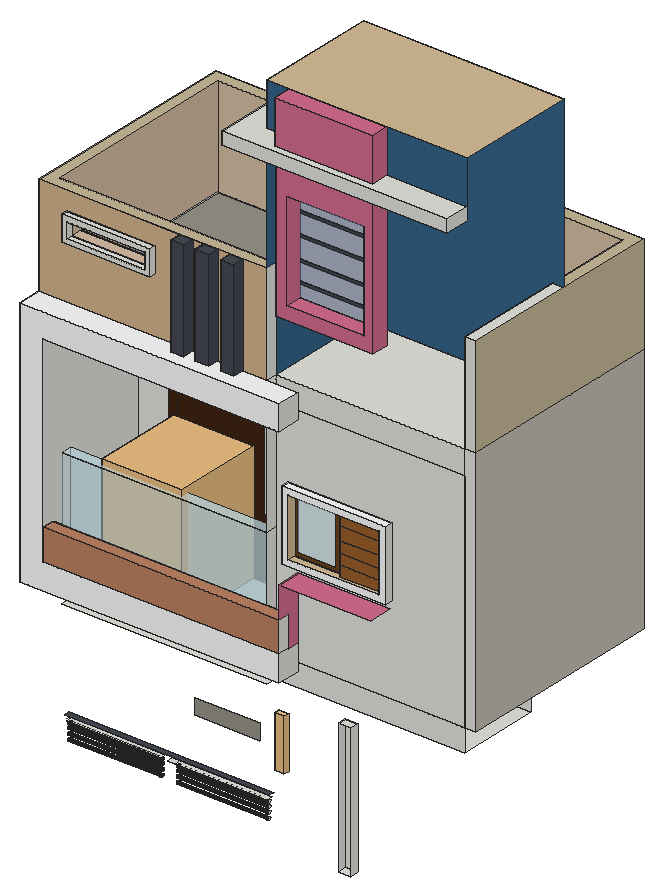
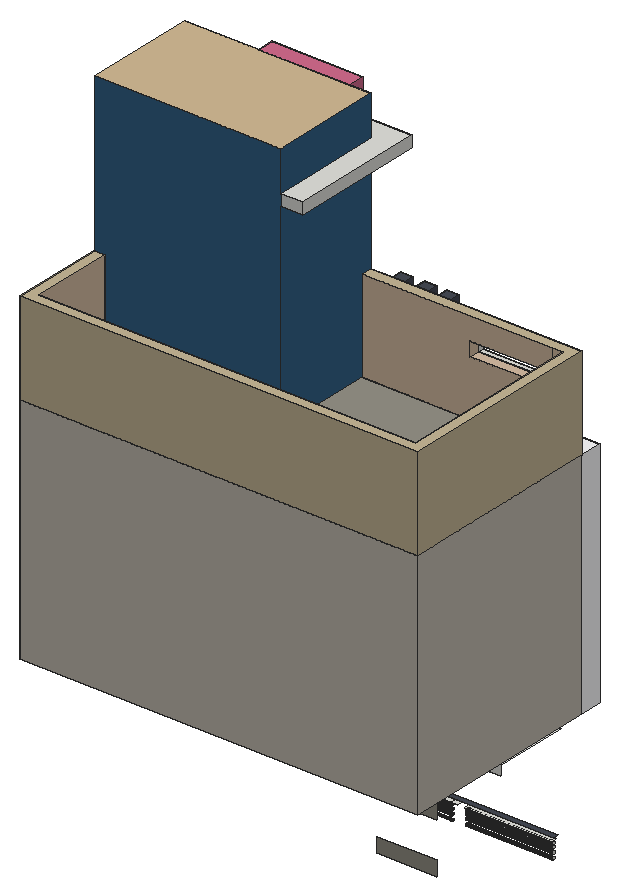
# SketchUp Ruby script. Lengths in inches.
U = 1.inch
M = Sketchup.active_model
def pt(a) = Geom::Point3d.new(a.map { |v| v * U })
def face(e, loops, mat)
  f = e.add_face(loops[0].map { |a| pt(a) })
  loops[1..].each { |l| e.add_face(l.map { |a| pt(a) }).erase! }
  f.material = f.back_material = mat if mat
  f
end
# faces: each face lists its corners as indices into pts; further lists are holes
def faces(e, pts, list, mat = nil) = list.each { |f| face(e, (f[0].is_a?(Array) ? f : [f]).map { |l| l.map { |i| pts[i] } }, mat) }
# xy, xz, yz: faces in a plane at the given z, y or x. An outline is a flat list of corners, or four numbers for a rectangle; further outlines are holes
def ring(l) = l.size == 4 ? [[l[0], l[1]], [l[2], l[1]], [l[2], l[3]], [l[0], l[3]]] : l.each_slice(2).to_a
def flat(e, list, mat, &to3) = list.each { |f| face(e, (f[0].is_a?(Array) ? f : [f]).map { |l| ring(l).map { |u, v| to3.(u, v) } }, mat) }
def xy(e, z, list, mat = nil) = flat(e, list, mat) { |x, y| [x, y, z] }
def xz(e, y, list, mat = nil) = flat(e, list, mat) { |x, z| [x, y, z] }
def yz(e, x, list, mat = nil) = flat(e, list, mat) { |y, z| [x, y, z] }
def lines(e, pts, list) = list.each { |a, b| e.add_line(pt(pts[a]), pt(pts[b])) }
# prism: a flat outline (further loops are holes) pulled along v
def prism(e, loops, v, mat = nil)
  f = face(e, loops, mat); d = Geom::Vector3d.new(v.map { |x| x * U })
  f.pushpull(f.normal.samedirection?(d) ? d.length : -d.length)
end
def box(e, o, s, mat = nil) = prism(e, [[o, [o[0] + s[0], o[1], o[2]], [o[0] + s[0], o[1] + s[1], o[2]], [o[0], o[1] + s[1], o[2]]]], [0, 0, s[2]], mat)
def at(x, y, z, deg = 0) = Geom::Transformation.translation(pt([x, y, z])) * Geom::Transformation.rotation(ORIGIN, Z_AXIS, deg.degrees)
def axes(o, x, y, z) = Geom::Transformation.new([*x, 0, *y, 0, *z, 0, *pt(o).to_a, 1])
def part(name) = M.definitions.add(name)
# library, detail: a bought-in or finely detailed component or shape, given as its bounding box
def library(name, o, s) = part(name).tap { |d| box(d.entities, o, s) }
def detail(e, o, s) = box(e.add_group.entities, o, s)
def put(e, d, t, mat = nil) = e.add_instance(d, t).tap { |i| i.material = mat if mat }
def group(e, t, mat = nil) = e.add_group.tap { |g| g.transformation = t; g.material = mat if mat }.entities
root = M.entities
M.materials.add("[0001_PaleVioletRed]").color = [211, 108, 142]
M.materials.add("[0035_Tan]").color = [210, 180, 140]
M.materials.add("[0100_SteelBlue]").color = [53, 99, 137]
M.materials.add("[Field Rectangle Tile]").color = [196, 189, 179]
M.materials.add("[Formica Beige]").color = [211, 187, 149]
M.materials.add("[Formica Graystone]").color = [149, 146, 135]
M.materials.add("[Formica Laminate Dark]").color = [70, 74, 84]
M.materials.add("[Formica Laminate Light]").color = [213, 189, 164]
M.materials.add("[Modern Siding]").color = [188, 130, 98]
M.materials.add("[Polished Concrete New]").color = [200, 200, 203]
M.materials.add("[Quartz Light Brown]").color = [199, 184, 152]
M.materials.add("[Quartz Light Grey]").color = [251, 251, 252]
M.materials.add("[Terrazzo Tile Light]").color = [219, 217, 210]
M.materials.add("[Translucent Glass Safety]").color = [204, 235, 244]
M.materials["[Translucent Glass Safety]"].alpha = 0.5
M.materials.add("[Translucent Glass Sky Reflection]").color = [126, 138, 183]
M.materials["[Translucent Glass Sky Reflection]"].alpha = 0.52
M.materials.add("[Window Covering 02]").color = [199, 178, 115]
M.materials.add("[Wood Cherry Original]").color = [96, 54, 26]
M.materials.add("[Wood Floor Dark]").color = [153, 94, 42]
M.materials.add("[Wood Floor Parquet]").color = [107, 65, 28]
M.materials.add("[Wood Veneer 01]").color = [63, 37, 19]
c1 = library("0 0 1",[0.77,0,0],[4.67,38.51,12])
c2 = library("chau cay",[-24.34,-109.24,0],[56.46,62.58,79.69])
xy(root,57.97,[[248.98,105.92,254.98,109.98]])
xy(root,67.58,[[108.27,118.87,153.22,121.64],[156.73,118.87,160.24,121.64],[160.24,118.87,204.4,121.64]])
xy(root,69.75,[[107.21,118.87,205.34,121.64]],"[Formica Laminate Dark]")
xy(root,118.16,[[107.21,117.35,107.21,162.72,296.05,162.72,296.05,122.78,205.34,122.78,205.34,117.35]])
xy(root,121.72,[[248.98,105.92,254.98,109.98]])
xy(root,129,[[96.16,105.92,101.58,117.35],[101.58,105.92,205.34,117.35],[205.34,105.92,220.625,117.35],[96.16,117.35,96.16,223.51,301.48,223.51,301.48,122.78,296.05,122.78,296.05,218.08,101.58,218.08,101.58,162.72,107.21,162.72,107.21,122.78,101.58,122.78,101.58,117.35],[101.58,117.35,205.34,122.78],
  [107.21,122.78,296.05,162.72],[101.58,162.72,296.05,170.43],[101.58,170.43,296.05,218.08]])
xy(root,141.375,[[107.21,105.92,220.625,111.64],[107.21,111.64,220.625,117.35],[107.21,117.35,205.34,122.78]])
xy(root,156.32,[[107.21,105.92,220.625,111.64]],"[Modern Siding]")
xy(root,162.92,[[195.11,162.72,264.3,170.43]])
xy(root,171.19,[[220.625,105.92,264.66,117.35]],"[0001_PaleVioletRed]")
xy(root,175.07,[[215.78,113.67,265.4,117.35]])
xy(root,178.04,[[241.96,115.6,262.43,117.35]])
xy(root,178.04,[[218.75,113.67,262.43,113.67,262.43,115.6,241.96,115.6,241.96,117.35,218.75,117.35]],"[Formica Beige]")
xy(root,183.1,[[241.96,115.6,262.43,117.35]])
xy(root,183.25,[[107.21,117.35,205.34,122.78]],"[Translucent Glass Safety]")
xy(root,188.16,[[241.96,115.6,262.43,117.35]])
xy(root,193.62,[[241.96,115.6,262.43,117.35]])
xy(root,199.79,[[241.96,115.6,262.43,117.35]])
xy(root,205.7,[[241.96,115.6,262.43,117.35]])
xy(root,205.7,[[218.75,113.67,218.75,117.35,241.96,117.35,241.96,115.6,262.43,115.6,262.43,113.67]],"[Formica Beige]")
xy(root,208.67,[[215.78,113.67,265.4,117.35]],"[Quartz Light Grey]")
xy(root,232.11,[[195.11,162.72,264.3,170.43]])
xy(root,237.17,[[107.21,105.92,205.34,117.35],[205.34,105.92,220.625,117.35],[107.21,117.35,205.34,122.78],[107.21,122.78,296.05,162.72]])
xy(root,239.2,[[101.58,170.43,296.05,218.08]])
xy(root,249,[[163.85,111.98,170.19,117.35],[175.41,111.98,181.76,117.35],[187.73,111.98,194.07,117.35],[96.16,117.35,96.16,223.51,301.48,223.51,301.48,122.78,296.05,122.78,296.05,218.08,101.58,218.08,101.58,117.35],[101.58,117.35,205.34,122.78],
  [205.34,122.78,296.05,175.59]])
xy(root,249,[[101.58,122.78,205.34,122.78,205.34,175.59,296.05,175.59,296.05,218.08,101.58,218.08]],"[Formica Graystone]")
xy(root,249,[[96.16,105.92,220.625,105.92,220.625,117.35,194.07,117.35,194.07,111.98,187.73,111.98,187.73,117.35,181.76,117.35,181.76,111.98,175.41,111.98,175.41,117.35,170.19,117.35,170.19,111.98,163.85,111.98,163.85,117.35,96.16,117.35]],"[Quartz Light Grey]")
xy(root,275.81,[[109.44,114.48,151.75,117.35]])
xy(root,278.13,[[111.77,114.48,149.43,117.35]])
xy(root,278.13,[[111.77,117.35,149.43,122.78]],"[Formica Laminate Light]")
xy(root,284.16,[[216.72,108.73,263.15,117.35]],"[0001_PaleVioletRed]")
xy(root,285.55,[[111.77,114.48,149.43,117.35]])
xy(root,285.55,[[111.77,117.35,149.43,122.78]],"[Formica Laminate Light]")
xy(root,287.87,[[109.44,114.48,151.75,117.35]])
xy(root,290.43,[[221.94,108.73,258.81,116.79]],"[0001_PaleVioletRed]")
xy(root,297,[[296.05,122.78,301.48,175.59]])
xy(root,297,[[163.85,111.98,170.19,117.35],[175.41,111.98,181.76,117.35],[187.73,111.98,194.07,117.35]],"[Formica Laminate Dark]")
xy(root,297,[[96.16,117.35,205.34,117.35,205.34,122.78,101.58,122.78,101.58,218.08,296.05,218.08,296.05,175.59,301.48,175.59,301.48,223.51,96.16,223.51]],"[Quartz Light Brown]")
xy(root,337.68,[[221.94,108.73,258.81,116.79]],"[0001_PaleVioletRed]")
xy(root,351.35,[[193.71,105.1,193.71,175.59,205.34,175.59,205.34,117.35,216.72,117.35,216.72,108.73,263.15,108.73,263.15,117.35,266.37,117.35,266.37,114.04,301.48,114.04,301.48,105.1],[216.72,108.73,263.15,117.35],[266.37,114.04,301.48,117.35]])
xy(root,357.29,[[193.71,105.1,301.48,105.1,301.48,117.35,263.15,117.35,263.15,108.73,216.08,108.73,216.08,117.35,205.34,117.35,205.34,175.59,193.71,175.59],[216.08,108.73,263.15,117.35]])
xy(root,378.0625,[[216.08,108.73,263.15,117.35]],"[0001_PaleVioletRed]")
xy(root,378.0625,[[205.34,117.35,301.48,175.59]],"[Formica Beige]")
xz(root,105.1,[[193.71,351.35,301.48,357.29]])
xz(root,105.92,[[107.21,141.375,220.625,156.32]],"[Modern Siding]")
xz(root,105.92,[[96.16,129,220.625,129,220.625,141.375,107.21,141.375,107.21,237.17,220.625,237.17,220.625,249,96.16,249]],"[Quartz Light Grey]")
xz(root,108.73,[[[216.72,284.16,263.15,351.35],[221.94,290.43,258.81,337.68]],[216.08,357.29,263.15,378.0625]],"[0001_PaleVioletRed]")
xz(root,109.98,[[248.98,57.97,254.98,121.72]])
xz(root,111.64,[[107.21,141.375,220.625,156.32]])
xz(root,111.98,[[163.85,249,170.19,297],[175.41,249,181.76,297],[187.73,249,194.07,297]],"[Formica Laminate Dark]")
xz(root,113.67,[[[215.78,175.07,265.4,208.67],[218.75,178.04,262.43,205.7]]],"[Quartz Light Grey]")
xz(root,114.48,[[[109.44,275.81,151.75,287.87],[111.77,278.13,149.43,285.55]]])
xz(root,115.6,[[241.96,178.04,262.43,183.1],[241.96,183.1,262.43,188.16],[241.96,188.16,262.43,193.62],[241.96,193.62,262.43,199.79],[241.96,199.79,262.43,205.7]],"[Wood Floor Dark]")
xz(root,116.79,[[221.94,296.5,258.81,297.76],[221.94,306.0625,258.81,307.32],[221.94,316.75,258.81,318.01],[221.94,327.125,258.81,328.38]],"[Formica Laminate Dark]")
xz(root,116.79,[[221.94,290.43,258.81,296.5],[221.94,297.76,258.81,306.0625],[221.94,307.32,258.81,316.75],[221.94,318.01,258.81,327.125],[221.94,328.38,258.81,337.68]],"[Translucent Glass Sky Reflection]")
xz(root,117.35,[[[215.78,175.07,265.4,208.67],[218.75,178.04,262.43,205.7]],[241.96,178.04,262.43,183.1],[241.96,183.1,262.43,188.16],[241.96,188.16,262.43,193.62],[241.96,193.62,262.43,199.79],
  [241.96,199.79,262.43,205.7],[163.85,249,170.19,297],[175.41,249,181.76,297],[187.73,249,194.07,297],[[109.44,275.81,151.75,287.87],[111.77,278.13,149.43,285.55]],
  [216.72,284.16,263.15,351.35],[216.08,357.29,263.15,378.0625]])
xz(root,117.35,[[[96.16,249,163.85,297],[109.44,275.81,151.75,287.87]],[170.19,249,175.41,297],[181.76,249,187.73,297],[194.07,249,205.34,297]],"[0035_Tan]")
xz(root,117.35,[[205.34,357.29,216.08,378.0625],[263.15,357.29,301.48,378.0625]],"[0100_SteelBlue]")
xz(root,117.35,[[240.59,178.04,241.96,205.7]],"[Formica Laminate Dark]")
xz(root,117.35,[[107.21,141.375,205.34,183.25],[220.59,179.88,238.75,203.85]],"[Translucent Glass Safety]")
xz(root,117.35,[[[218.75,178.04,240.59,205.7],[220.59,179.88,238.75,203.85]]],"[Wood Floor Parquet]")
xz(root,122.78,[[205.34,118.16,296.05,129],[107.21,129,205.34,141.375],[205.34,129,296.05,237.17],[296.05,129,301.48,249],[107.21,237.17,205.34,249],
  [205.34,237.17,296.05,249],[296.05,249,301.48,297]])
xz(root,122.78,[[101.58,249,107.21,297],[[107.21,249,205.34,297],[111.77,278.13,149.43,285.55]]],"[Formica Laminate Light]")
xz(root,122.78,[[107.21,141.375,205.34,183.25]],"[Translucent Glass Safety]")
xz(root,162.72,[[101.58,118.16,296.05,129],[[107.21,129,121.5625,129,121.5625,232.125,181,232.125,181,129,296.05,129,296.05,237.17,107.21,237.17],[195.11,162.92,264.3,232.11]]])
xz(root,162.72,[[134.59,60.26,166.02,67.7],[134.59,86.26,166.02,93.7],[131.36,156.37,163.17,163.24],[131.36,178.99,163.17,185.87],[131.36,202.49,163.17,209.37]],"[Formica Graystone]")
xz(root,162.72,[[167.92,157.88,170.35,202.19]],"[Terrazzo Tile Light]")
xz(root,162.72,[[199.8,167.62,226.2,227.42],[230.11,167.62,259.61,227.42]],"[Window Covering 02]")
xz(root,162.72,[[[195.11,162.92,264.3,232.11],[199.8,167.62,259.61,227.42]],[226.2,167.62,230.11,227.42]],"[Wood Cherry Original]")
xz(root,162.72,[[[121.5625,129,181,232.125],[126.22,133.65,176.35,227.47]],[[126.22,133.65,176.35,227.47],[131.36,202.49,163.17,209.37],[131.36,156.37,163.17,163.24],[131.36,178.99,163.17,185.87],[167.92,157.88,170.35,202.19]]],"[Wood Veneer 01]")
xz(root,170.43,[[[101.58,129,296.05,239.2],[195.11,162.92,264.3,232.11]]])
xz(root,175.59,[[193.71,351.35,205.34,357.29]])
xz(root,175.59,[[205.34,249,205.34,378.0625,301.48,378.0625,301.48,297,296.05,297,296.05,249]],"[0100_SteelBlue]")
xz(root,218.08,[[101.58,129,296.05,239.2],[101.58,239.2,296.05,249]])
xz(root,218.08,[[101.58,249,296.05,297]],"[Formica Laminate Light]")
xz(root,223.51,[[96.16,129,301.48,249]],"[Field Rectangle Tile]")
xz(root,223.51,[[96.16,249,301.48,297]],"[Quartz Light Brown]")
yz(root,96.16,[[117.35,129,223.51,249]],"[Field Rectangle Tile]")
yz(root,96.16,[[117.35,249,223.51,297]],"[Quartz Light Brown]")
yz(root,96.16,[[105.92,129,117.35,249]],"[Quartz Light Grey]")
yz(root,101.58,[[162.72,129,170.43,249],[170.43,129,218.08,239.2],[170.43,239.2,218.08,249]])
yz(root,101.58,[[122.78,249,218.08,297]],"[Formica Laminate Light]")
yz(root,107.21,[[122.78,129,162.72,129,162.72,237.17,105.92,237.17,105.92,156.32,111.64,156.32,111.64,141.375,117.35,141.375,117.35,183.25,122.78,183.25],[105.92,141.375,111.64,156.32],[117.35,141.375,122.78,183.25]])
yz(root,108.27,[[120.22,58.6,120.06,58.62,119.91,58.68,119.78,58.78,119.68,58.91,119.61,59.0625,119.59,59.22,119.61,59.38,119.68,59.54,119.78,59.66,119.91,59.76,120.06,59.83,120.22,59.85,120.38,59.83,120.53,59.76,120.66,59.66,120.76,59.54,120.82,59.38,120.84,59.22,120.82,59.0625,120.76,58.91,120.66,58.78,120.53,58.68,120.38,58.62],[120.22,61.16,120.06,61.18,119.91,61.24,119.78,61.34,119.68,61.47,119.61,61.625,119.59,61.79,119.61,61.95,119.68,62.1,119.78,62.23,119.91,62.33,120.06,62.39,120.22,62.41,120.38,62.39,120.53,62.33,120.66,62.23,120.76,62.1,120.82,61.95,120.84,61.79,120.82,61.625,120.76,61.47,120.66,61.34,120.53,61.24,120.38,61.18],[120.22,63.72,120.06,63.74,119.91,63.81,119.78,63.91,119.68,64.04,119.61,64.1875,119.59,64.35,119.61,64.51,119.68,64.66,119.78,64.79,119.91,64.89,120.06,64.95,120.22,64.97,120.38,64.95,120.53,64.89,120.66,64.79,120.76,64.66,120.82,64.51,120.84,64.35,120.82,64.1875,120.76,64.04,120.66,63.91,120.53,63.81,120.38,63.74],[120.22,65.6,120.06,65.62,119.91,65.68,119.78,65.78,119.68,65.91,119.61,66.0625,119.59,66.22,119.61,66.38,119.68,66.54,119.78,66.66,119.91,66.76,120.06,66.83,120.22,66.85,120.38,66.83,120.53,66.76,120.66,66.66,120.76,66.54,120.82,66.38,120.84,66.22,120.82,66.0625,120.76,65.91,120.66,65.78,120.53,65.68,120.38,65.62]])
yz(root,109.44,[[114.48,275.81,117.35,287.87]])
yz(root,111.77,[[114.48,278.13,117.35,285.55]])
yz(root,111.77,[[117.35,278.13,122.78,285.55]],"[Formica Laminate Light]")
yz(root,149.43,[[114.48,278.13,117.35,285.55]])
yz(root,149.43,[[117.35,278.13,122.78,285.55]],"[Formica Laminate Light]")
yz(root,151.75,[[114.48,275.81,117.35,287.87]])
yz(root,163.85,[[111.98,249,117.35,297]],"[Formica Laminate Dark]")
yz(root,170.19,[[111.98,249,117.35,297]],"[Formica Laminate Dark]")
yz(root,175.41,[[111.98,249,117.35,297]],"[Formica Laminate Dark]")
yz(root,181.76,[[111.98,249,117.35,297]],"[Formica Laminate Dark]")
yz(root,187.73,[[111.98,249,117.35,297]],"[Formica Laminate Dark]")
yz(root,193.71,[[105.1,351.35,175.59,357.29]])
yz(root,194.07,[[111.98,249,117.35,297]],"[Formica Laminate Dark]")
yz(root,195.11,[[162.72,162.92,170.43,232.11]])
yz(root,204.4,[[120.29,58.16,120.45,58.1875,120.6,58.25,120.73,58.35,120.83,58.48,120.89,58.63,120.91,58.79,120.89,58.95,120.83,59.1,120.73,59.23,120.6,59.33,120.45,59.39,120.29,59.41,120.13,59.39,119.98,59.33,119.85,59.23,119.75,59.1,119.6875,58.95,119.66,58.79,119.6875,58.63,119.75,58.48,119.85,58.35,119.98,58.25,120.13,58.1875],[120.29,60.85,120.45,60.875,120.6,60.9375,120.73,61.04,120.83,61.16,120.89,61.32,120.91,61.48,120.89,61.64,120.83,61.79,120.73,61.92,120.6,62.02,120.45,62.08,120.29,62.1,120.13,62.08,119.98,62.02,119.85,61.92,119.75,61.79,119.6875,61.64,119.66,61.48,119.6875,61.32,119.75,61.16,119.85,61.04,119.98,60.9375,120.13,60.875],[120.29,63.23,120.45,63.25,120.6,63.3125,120.73,63.41,120.83,63.54,120.89,63.69,120.91,63.85,120.89,64.01,120.83,64.16,120.73,64.29,120.6,64.39,120.45,64.46,120.29,64.48,120.13,64.46,119.98,64.39,119.85,64.29,119.75,64.16,119.6875,64.01,119.66,63.85,119.6875,63.69,119.75,63.54,119.85,63.41,119.98,63.3125,120.13,63.25],[120.29,65.54,120.45,65.5625,120.6,65.625,120.73,65.72,120.83,65.85,120.89,66,120.91,66.16,120.89,66.33,120.83,66.48,120.73,66.61,120.6,66.71,120.45,66.77,120.29,66.79,120.13,66.77,119.98,66.71,119.85,66.61,119.75,66.48,119.6875,66.33,119.66,66.16,119.6875,66,119.75,65.85,119.85,65.72,119.98,65.625,120.13,65.5625]])
yz(root,205.34,[[117.35,141.375,122.78,183.25],[117.35,183.25,122.78,237.17],[117.35,249,122.78,297]])
yz(root,205.34,[[122.78,249,122.78,297,117.35,297,117.35,351.35,175.59,351.35,175.59,249],[117.35,357.29,175.59,378.0625]],"[0100_SteelBlue]")
yz(root,215.78,[[113.67,175.07,117.35,208.67]],"[Quartz Light Grey]")
yz(root,216.08,[[108.73,357.29,117.35,378.0625]],"[0001_PaleVioletRed]")
yz(root,216.72,[[108.73,284.16,117.35,351.35]],"[0001_PaleVioletRed]")
yz(root,218.75,[[113.67,178.04,117.35,205.7]],"[Formica Beige]")
yz(root,220.625,[[105.92,129,117.35,141.375],[105.92,141.375,111.64,156.32],[105.92,237.17,117.35,249]])
yz(root,220.625,[[111.64,141.375,111.64,156.32,105.92,156.32,105.92,171.19,117.35,171.19,117.35,141.375]],"[0001_PaleVioletRed]")
yz(root,221.94,[[108.73,290.43,116.79,337.68]],"[0001_PaleVioletRed]")
yz(root,241.96,[[115.6,178.04,117.35,183.1],[115.6,183.1,117.35,188.16],[115.6,188.16,117.35,193.62],[115.6,193.62,117.35,199.79],[115.6,199.79,117.35,205.7]],"[Wood Floor Dark]")
yz(root,248.98,[[105.92,57.97,109.98,121.72]])
yz(root,254.98,[[105.92,57.97,109.98,121.72]])
yz(root,258.81,[[108.73,290.43,116.79,337.68]],"[0001_PaleVioletRed]")
yz(root,262.43,[[115.6,178.04,117.35,183.1],[115.6,183.1,117.35,188.16],[115.6,188.16,117.35,193.62],[115.6,193.62,117.35,199.79],[115.6,199.79,117.35,205.7]])
yz(root,262.43,[[113.67,178.04,115.6,205.7]],"[Formica Beige]")
yz(root,263.15,[[108.73,284.16,117.35,351.35],[108.73,357.29,117.35,378.0625]],"[0001_PaleVioletRed]")
yz(root,264.3,[[162.72,162.92,170.43,232.11]])
yz(root,265.4,[[113.67,175.07,117.35,208.67]])
yz(root,296.05,[[122.78,129,162.72,237.17],[162.72,129,170.43,249],[170.43,129,218.08,239.2],[122.78,249,175.59,297]])
yz(root,296.05,[[175.59,249,218.08,297]],"[Formica Laminate Light]")
yz(root,301.48,[[105.1,351.35,117.35,357.29]])
yz(root,301.48,[[122.78,129,223.51,249]],"[Field Rectangle Tile]")
yz(root,301.48,[[122.78,249,223.51,297]],"[Quartz Light Brown]")
p = [[204.4,119.98,58.25],[204.4,119.85,58.35],[160.24,119.85,58.35],[160.24,119.98,58.25],[204.4,120.13,58.1875],[160.24,120.13,58.1875],
  [204.4,120.29,58.16],[160.24,120.29,58.16],[204.4,120.45,58.1875],[160.24,120.45,58.1875],[204.4,120.6,58.25],[160.24,120.6,58.25],
  [204.4,120.73,58.35],[160.24,120.73,58.35],[204.4,119.75,58.48],[160.24,119.75,58.48],[204.4,120.83,58.48],[160.24,120.83,58.48],
  [204.4,119.6875,58.63],[160.24,119.6875,58.63],[204.4,120.89,58.63],[160.24,120.89,58.63],[204.4,119.66,58.79],[160.24,119.66,58.79],
  [108.27,119.91,58.68],[108.27,120.06,58.62],[153.22,120.06,58.62],[153.22,119.91,58.68],[108.27,120.22,58.6],[153.22,120.22,58.6],
  [108.27,120.38,58.62],[153.22,120.38,58.62],[108.27,120.53,58.68],[153.22,120.53,58.68],[204.4,120.91,58.79],[160.24,120.91,58.79],
  [108.27,119.78,58.78],[153.22,119.78,58.78],[108.27,120.66,58.78],[153.22,120.66,58.78],[108.27,119.68,58.91],[153.22,119.68,58.91],
  [204.4,119.6875,58.95],[160.24,119.6875,58.95],[108.27,120.76,58.91],[153.22,120.76,58.91],[204.4,120.89,58.95],[160.24,120.89,58.95],
  [108.27,119.61,59.0625],[153.22,119.61,59.0625],[108.27,120.82,59.0625],[153.22,120.82,59.0625],[204.4,119.75,59.1],[160.24,119.75,59.1],
  [204.4,120.83,59.1],[160.24,120.83,59.1],[108.27,119.59,59.22],[153.22,119.59,59.22],[204.4,119.85,59.23],[160.24,119.85,59.23],
  [204.4,120.73,59.23],[160.24,120.73,59.23],[108.27,120.84,59.22],[153.22,120.84,59.22],[108.27,119.61,59.38],[153.22,119.61,59.38],
  [204.4,119.98,59.33],[160.24,119.98,59.33],[204.4,120.6,59.33],[160.24,120.6,59.33],[108.27,120.82,59.38],[153.22,120.82,59.38],
  [204.4,120.13,59.39],[160.24,120.13,59.39],[204.4,120.45,59.39],[160.24,120.45,59.39],[108.27,119.68,59.54],[153.22,119.68,59.54],
  [204.4,120.29,59.41],[160.24,120.29,59.41],[108.27,120.76,59.54],[153.22,120.76,59.54],[108.27,119.78,59.66],[153.22,119.78,59.66],
  [108.27,120.66,59.66],[153.22,120.66,59.66],[108.27,119.91,59.76],[153.22,119.91,59.76],[108.27,120.53,59.76],[153.22,120.53,59.76],
  [108.27,120.06,59.83],[153.22,120.06,59.83],[108.27,120.22,59.85],[153.22,120.22,59.85],[108.27,120.38,59.83],[153.22,120.38,59.83],
  [204.4,119.98,60.9375],[204.4,119.85,61.04],[160.24,119.85,61.04],[160.24,119.98,60.9375],[204.4,120.13,60.875],[160.24,120.13,60.875],
  [204.4,120.29,60.85],[160.24,120.29,60.85],[204.4,120.45,60.875],[160.24,120.45,60.875],[204.4,120.6,60.9375],[160.24,120.6,60.9375],
  [204.4,120.73,61.04],[160.24,120.73,61.04],[204.4,119.75,61.16],[160.24,119.75,61.16],[204.4,120.83,61.16],[160.24,120.83,61.16],
  [204.4,119.6875,61.32],[160.24,119.6875,61.32],[108.27,119.78,61.34],[108.27,119.91,61.24],[153.22,119.91,61.24],[153.22,119.78,61.34],
  [108.27,120.06,61.18],[153.22,120.06,61.18],[108.27,120.22,61.16],[153.22,120.22,61.16],[108.27,120.38,61.18],[153.22,120.38,61.18],
  [108.27,120.53,61.24],[153.22,120.53,61.24],[108.27,120.66,61.34],[153.22,120.66,61.34],[204.4,120.89,61.32],[160.24,120.89,61.32],
  [108.27,119.68,61.47],[153.22,119.68,61.47],[204.4,119.66,61.48],[160.24,119.66,61.48],[108.27,120.76,61.47],[153.22,120.76,61.47],
  [204.4,120.91,61.48],[160.24,120.91,61.48],[108.27,119.61,61.625],[153.22,119.61,61.625],[204.4,119.6875,61.64],[160.24,119.6875,61.64],
  [108.27,120.82,61.625],[153.22,120.82,61.625],[204.4,120.89,61.64],[160.24,120.89,61.64],[108.27,119.59,61.79],[153.22,119.59,61.79],
  [204.4,119.75,61.79],[160.24,119.75,61.79],[108.27,120.84,61.79],[153.22,120.84,61.79],[204.4,120.83,61.79],[160.24,120.83,61.79],
  [108.27,119.61,61.95],[153.22,119.61,61.95],[204.4,119.85,61.92],[160.24,119.85,61.92],[204.4,120.73,61.92],[160.24,120.73,61.92],
  [108.27,120.82,61.95],[153.22,120.82,61.95],[108.27,119.68,62.1],[153.22,119.68,62.1],[204.4,119.98,62.02],[160.24,119.98,62.02],
  [204.4,120.6,62.02],[160.24,120.6,62.02],[108.27,120.76,62.1],[153.22,120.76,62.1],[204.4,120.13,62.08],[160.24,120.13,62.08],
  [204.4,120.45,62.08],[160.24,120.45,62.08],[108.27,119.78,62.23],[153.22,119.78,62.23],[204.4,120.29,62.1],[160.24,120.29,62.1],
  [108.27,120.66,62.23],[153.22,120.66,62.23],[108.27,119.91,62.33],[153.22,119.91,62.33],[108.27,120.53,62.33],[153.22,120.53,62.33],
  [108.27,120.06,62.39],[153.22,120.06,62.39],[108.27,120.38,62.39],[153.22,120.38,62.39],[108.27,120.22,62.41],[153.22,120.22,62.41],
  [204.4,120.13,63.25],[204.4,119.98,63.3125],[160.24,119.98,63.3125],[160.24,120.13,63.25],[204.4,120.29,63.23],[160.24,120.29,63.23],
  [204.4,120.45,63.25],[160.24,120.45,63.25],[204.4,120.6,63.3125],[160.24,120.6,63.3125],[204.4,119.85,63.41],[160.24,119.85,63.41],
  [204.4,120.73,63.41],[160.24,120.73,63.41],[204.4,119.75,63.54],[160.24,119.75,63.54],[204.4,120.83,63.54],[160.24,120.83,63.54],
  [204.4,119.6875,63.69],[160.24,119.6875,63.69],[204.4,120.89,63.69],[160.24,120.89,63.69],[204.4,119.66,63.85],[160.24,119.66,63.85],
  [108.27,119.91,63.81],[108.27,120.06,63.74],[153.22,120.06,63.74],[153.22,119.91,63.81],[108.27,120.22,63.72],[153.22,120.22,63.72],
  [108.27,120.38,63.74],[153.22,120.38,63.74],[108.27,120.53,63.81],[153.22,120.53,63.81],[204.4,120.91,63.85],[160.24,120.91,63.85],
  [108.27,119.78,63.91],[153.22,119.78,63.91],[108.27,120.66,63.91],[153.22,120.66,63.91],[108.27,119.68,64.04],[153.22,119.68,64.04],
  [204.4,119.6875,64.01],[160.24,119.6875,64.01],[108.27,120.76,64.04],[153.22,120.76,64.04],[204.4,120.89,64.01],[160.24,120.89,64.01],
  [108.27,119.61,64.1875],[153.22,119.61,64.1875],[204.4,119.75,64.16],[160.24,119.75,64.16],[108.27,120.82,64.1875],[153.22,120.82,64.1875],
  [204.4,120.83,64.16],[160.24,120.83,64.16],[108.27,119.59,64.35],[153.22,119.59,64.35],[204.4,119.85,64.29],[160.24,119.85,64.29],
  [204.4,120.73,64.29],[160.24,120.73,64.29],[108.27,120.84,64.35],[153.22,120.84,64.35],[108.27,119.61,64.51],[153.22,119.61,64.51],
  [204.4,119.98,64.39],[160.24,119.98,64.39],[204.4,120.6,64.39],[160.24,120.6,64.39],[108.27,120.82,64.51],[153.22,120.82,64.51],
  [204.4,120.13,64.46],[160.24,120.13,64.46],[204.4,120.45,64.46],[160.24,120.45,64.46],[108.27,119.68,64.66],[153.22,119.68,64.66],
  [204.4,120.29,64.48],[160.24,120.29,64.48],[108.27,120.76,64.66],[153.22,120.76,64.66],[108.27,119.78,64.79],[153.22,119.78,64.79],
  [108.27,120.66,64.79],[153.22,120.66,64.79],[108.27,119.91,64.89],[153.22,119.91,64.89],[108.27,120.53,64.89],[153.22,120.53,64.89],
  [108.27,120.06,64.95],[153.22,120.06,64.95],[108.27,120.38,64.95],[153.22,120.38,64.95],[108.27,120.22,64.97],[153.22,120.22,64.97],
  [204.4,120.29,65.54],[204.4,120.13,65.5625],[160.24,120.13,65.5625],[160.24,120.29,65.54],[204.4,120.45,65.5625],[160.24,120.45,65.5625],
  [204.4,119.98,65.625],[204.4,119.85,65.72],[160.24,119.85,65.72],[160.24,119.98,65.625],[108.27,119.91,65.68],[108.27,120.06,65.62],
  [153.22,120.06,65.62],[153.22,119.91,65.68],[108.27,120.22,65.6],[153.22,120.22,65.6],[108.27,120.38,65.62],[153.22,120.38,65.62],
  [108.27,120.53,65.68],[153.22,120.53,65.68],[204.4,120.6,65.625],[160.24,120.6,65.625],[204.4,120.73,65.72],[160.24,120.73,65.72],
  [204.4,119.75,65.85],[160.24,119.75,65.85],[108.27,119.78,65.78],[153.22,119.78,65.78],[108.27,120.66,65.78],[153.22,120.66,65.78],
  [204.4,120.83,65.85],[160.24,120.83,65.85],[108.27,119.68,65.91],[153.22,119.68,65.91],[108.27,120.76,65.91],[153.22,120.76,65.91],
  [108.27,119.61,66.0625],[153.22,119.61,66.0625],[204.4,119.6875,66],[160.24,119.6875,66],[108.27,120.82,66.0625],[153.22,120.82,66.0625],
  [204.4,120.89,66],[160.24,120.89,66],[204.4,119.66,66.16],[160.24,119.66,66.16],[204.4,120.91,66.16],[160.24,120.91,66.16],
  [108.27,119.59,66.22],[153.22,119.59,66.22],[108.27,120.84,66.22],[153.22,120.84,66.22],[108.27,119.61,66.38],[153.22,119.61,66.38],
  [204.4,119.6875,66.33],[160.24,119.6875,66.33],[108.27,120.82,66.38],[153.22,120.82,66.38],[204.4,120.89,66.33],[160.24,120.89,66.33],
  [204.4,119.75,66.48],[160.24,119.75,66.48],[204.4,120.83,66.48],[160.24,120.83,66.48],[108.27,119.68,66.54],[153.22,119.68,66.54],
  [108.27,120.76,66.54],[153.22,120.76,66.54],[108.27,119.78,66.66],[153.22,119.78,66.66],[204.4,119.85,66.61],[160.24,119.85,66.61],
  [108.27,120.66,66.66],[153.22,120.66,66.66],[204.4,120.73,66.61],[160.24,120.73,66.61],[204.4,119.98,66.71],[160.24,119.98,66.71],
  [204.4,120.6,66.71],[160.24,120.6,66.71],[108.27,119.91,66.76],[153.22,119.91,66.76],[204.4,120.13,66.77],[160.24,120.13,66.77],
  [108.27,120.53,66.76],[153.22,120.53,66.76],[204.4,120.45,66.77],[160.24,120.45,66.77],[108.27,120.06,66.83],[153.22,120.06,66.83],
  [108.27,120.22,66.85],[153.22,120.22,66.85],[204.4,120.29,66.79],[160.24,120.29,66.79],[108.27,120.38,66.83],[153.22,120.38,66.83],
  [107.21,162.72,237.17],[107.21,162.72,249],[108.27,118.87,68.58],[108.27,121.64,68.58]]
faces(root,p,[[0,1,2,3],[4,0,3,5],[6,4,5,7],[8,6,7,9],[10,8,9,11],[12,10,11,13],[1,14,15,2],[16,12,13,17],
  [14,18,19,15],[20,16,17,21],[18,22,23,19],[24,25,26,27],[25,28,29,26],[28,30,31,29],[30,32,33,31],[34,20,21,35],
  [36,24,27,37],[32,38,39,33],[40,36,37,41],[22,42,43,23],[38,44,45,39],[46,34,35,47],[48,40,41,49],[44,50,51,45],
  [42,52,53,43],[54,46,47,55],[56,48,49,57],[52,58,59,53],[60,54,55,61],[50,62,63,51],[64,56,57,65],[58,66,67,59],
  [68,60,61,69],[62,70,71,63],[66,72,73,67],[74,68,69,75],[76,64,65,77],[72,78,79,73],[78,74,75,79],[70,80,81,71],
  [82,76,77,83],[80,84,85,81],[86,82,83,87],[84,88,89,85],[90,86,87,91],[92,90,91,93],[94,92,93,95],[88,94,95,89],
  [96,97,98,99],[100,96,99,101],[102,100,101,103],[104,102,103,105],[106,104,105,107],[108,106,107,109],[97,110,111,98],[112,108,109,113],
  [110,114,115,111],[116,117,118,119],[117,120,121,118],[120,122,123,121],[122,124,125,123],[124,126,127,125],[126,128,129,127],[130,112,113,131],
  [132,116,119,133],[114,134,135,115],[128,136,137,129],[138,130,131,139],[140,132,133,141],[134,142,143,135],[136,144,145,137],[146,138,139,147],
  [148,140,141,149],[142,150,151,143],[144,152,153,145],[154,146,147,155],[156,148,149,157],[150,158,159,151],[160,154,155,161],[152,162,163,153],
  [164,156,157,165],[158,166,167,159],[168,160,161,169],[162,170,171,163],[166,172,173,167],[174,168,169,175],[176,164,165,177],[172,178,179,173],
  [178,174,175,179],[170,180,181,171],[182,176,177,183],[180,184,185,181],[186,182,183,187],[184,188,189,185],[190,186,187,191],[188,190,191,189],
  [192,193,194,195],[196,192,195,197],[198,196,197,199],[200,198,199,201],[193,202,203,194],[204,200,201,205],[202,206,207,203],[208,204,205,209],
  [206,210,211,207],[212,208,209,213],[210,214,215,211],[216,217,218,219],[217,220,221,218],[220,222,223,221],[222,224,225,223],[226,212,213,227],
  [228,216,219,229],[224,230,231,225],[232,228,229,233],[214,234,235,215],[230,236,237,231],[238,226,227,239],[240,232,233,241],[234,242,243,235],
  [236,244,245,237],[246,238,239,247],[248,240,241,249],[242,250,251,243],[252,246,247,253],[244,254,255,245],[256,248,249,257],[250,258,259,251],
  [260,252,253,261],[254,262,263,255],[258,264,265,259],[266,260,261,267],[268,256,257,269],[264,270,271,265],[270,266,267,271],[262,272,273,263],
  [274,268,269,275],[272,276,277,273],[278,274,275,279],[276,280,281,277],[282,278,279,283],[280,284,285,281],[286,282,283,287],[284,286,287,285],
  [288,289,290,291],[292,288,291,293],[294,295,296,297],[298,299,300,301],[289,294,297,290],[299,302,303,300],[302,304,305,303],[304,306,307,305],
  [308,292,293,309],[310,308,309,311],[295,312,313,296],[314,298,301,315],[306,316,317,307],[318,310,311,319],[320,314,315,321],[316,322,323,317],
  [324,320,321,325],[312,326,327,313],[322,328,329,323],[330,318,319,331],[326,332,333,327],[334,330,331,335],[336,324,325,337],[328,338,339,329],
  [340,336,337,341],[332,342,343,333],[338,344,345,339],[346,334,335,347],[342,348,349,343],[350,346,347,351],[352,340,341,353],[344,354,355,345],
  [356,352,353,357],[348,358,359,349],[354,360,361,355],[362,350,351,363],[358,364,365,359],[366,362,363,367],[368,356,357,369],[364,370,371,365],
  [360,372,373,361],[374,366,367,375],[376,368,369,377],[378,376,377,379],[370,380,381,371],[382,378,379,383],[380,374,375,381],[372,382,383,373]],"[Polished Concrete New]")
lines(root,p,[[384,385],[386,387]])
put(root,c1,axes([210.58,117.35,84.39],[1,0,0],[0,0,0.646],[0,-0.22,0]))
put(root,c2,axes([141.2,195.06,129],[0.68423,0,0],[0,0.693,0],[0,0,0.71359]))
